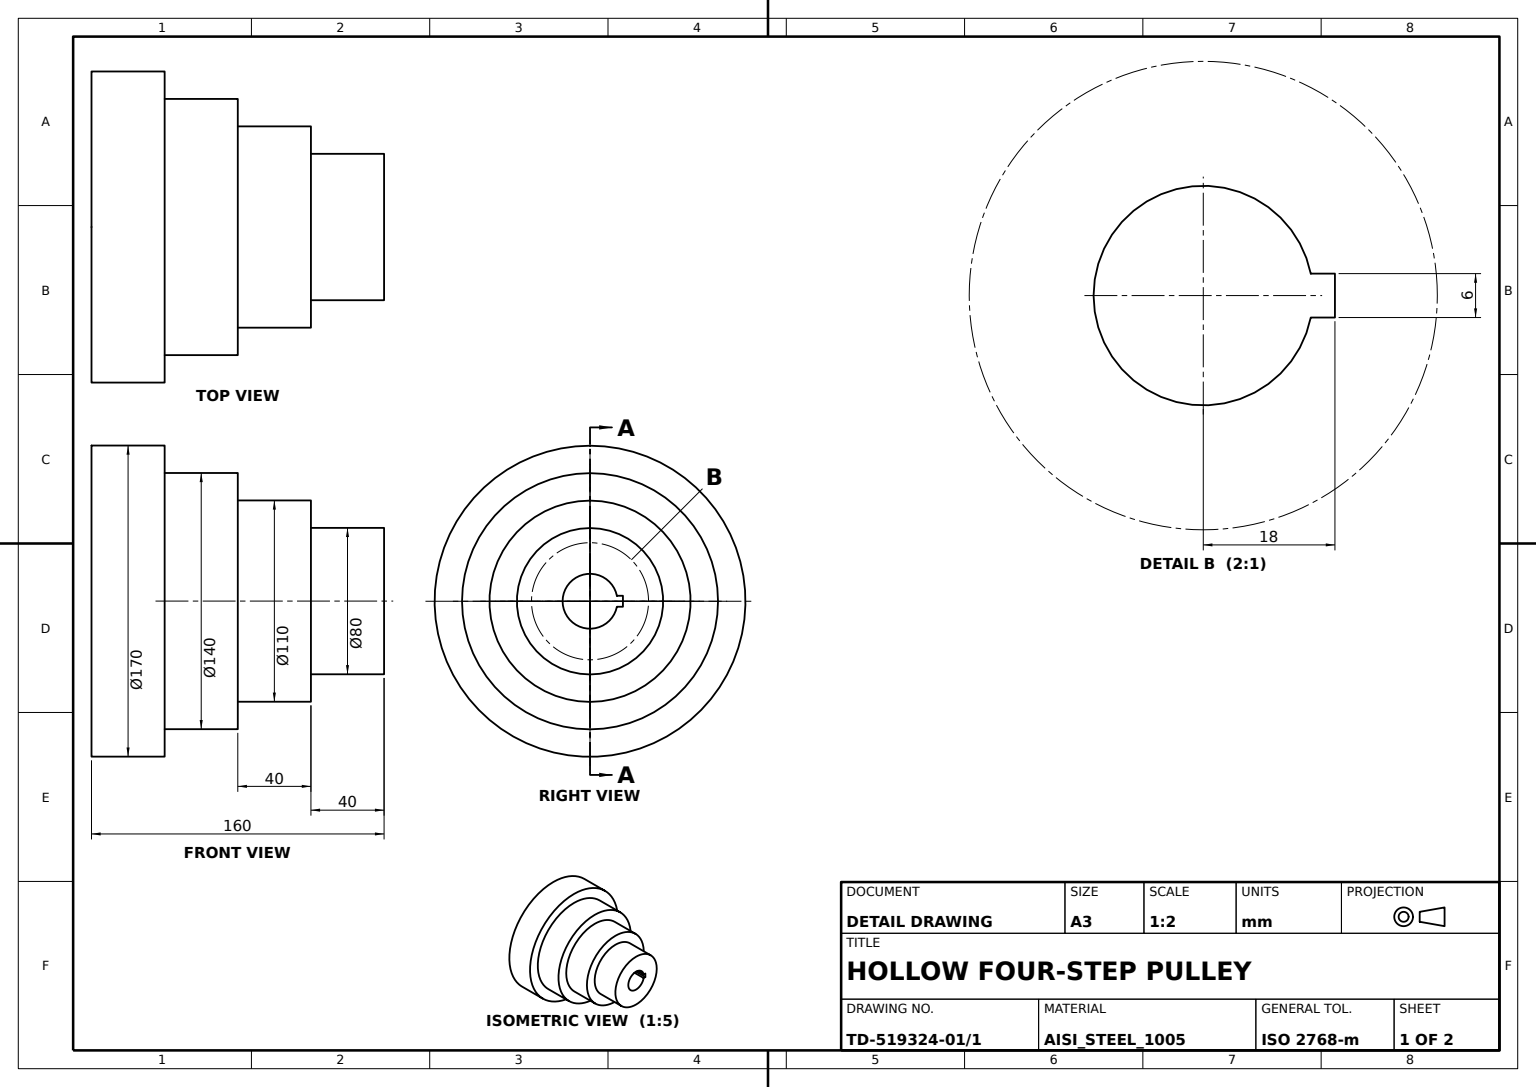
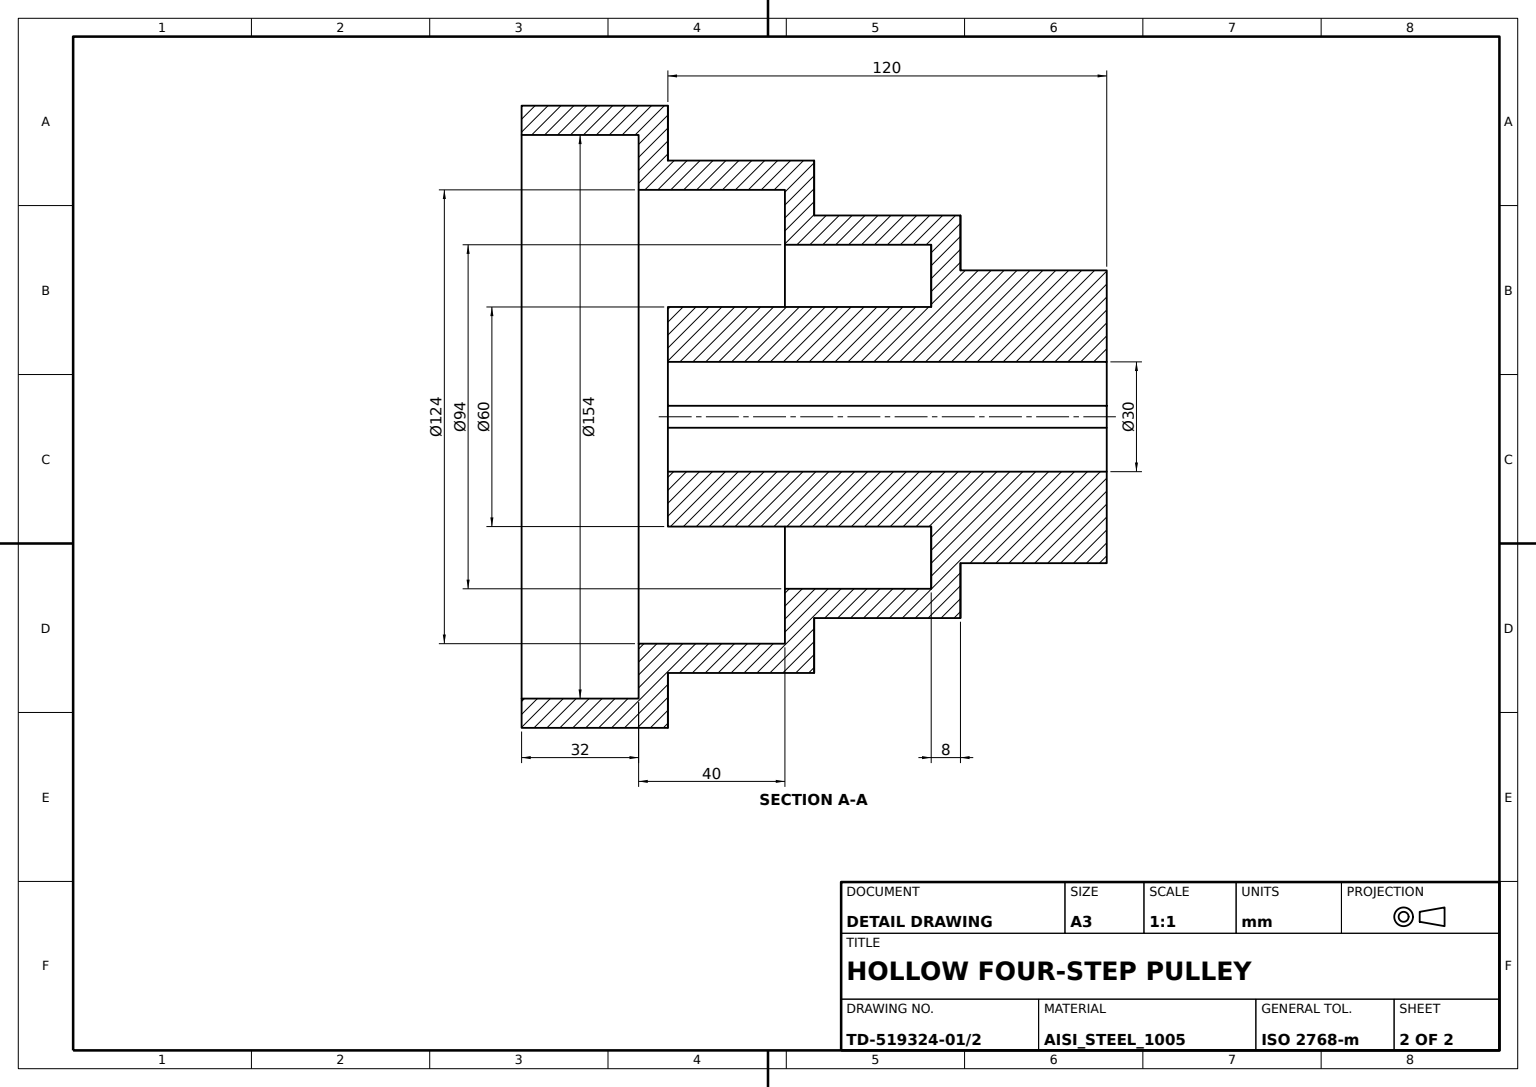
ISO-10303-21;
HEADER;
FILE_DESCRIPTION((''),'2;1');
FILE_NAME('','',(''),(''),'','','');
FILE_SCHEMA(('AUTOMOTIVE_DESIGN'));
ENDSEC;
DATA;
#1=APPLICATION_CONTEXT('');
#2=PRODUCT_CONTEXT('',#1,'mechanical');
#3=PRODUCT('','','',(#2));
#4=PRODUCT_DEFINITION_FORMATION('','',#3);
#5=PRODUCT_DEFINITION_CONTEXT('',#1,'design');
#6=PRODUCT_DEFINITION('','',#4,#5);
#7=PRODUCT_DEFINITION_SHAPE('','',#6);
#8=(LENGTH_UNIT()NAMED_UNIT(*)SI_UNIT(.MILLI.,.METRE.));
#9=(NAMED_UNIT(*)PLANE_ANGLE_UNIT()SI_UNIT($,.RADIAN.));
#10=(NAMED_UNIT(*)SI_UNIT($,.STERADIAN.)SOLID_ANGLE_UNIT());
#11=UNCERTAINTY_MEASURE_WITH_UNIT(LENGTH_MEASURE(0.005),#8,'distance_accuracy_value','');
#12=(GEOMETRIC_REPRESENTATION_CONTEXT(3)GLOBAL_UNCERTAINTY_ASSIGNED_CONTEXT((#11))GLOBAL_UNIT_ASSIGNED_CONTEXT((#8,#9,#10))REPRESENTATION_CONTEXT('',''));
#13=CARTESIAN_POINT('',(0.,72.,62.));
#14=VERTEX_POINT('',#13);
#15=CARTESIAN_POINT('',(0.,72.,0.));
#16=DIRECTION('',(0.,1.,0.));
#17=DIRECTION('',(0.,0.,1.));
#18=AXIS2_PLACEMENT_3D('',#15,#16,#17);
#19=CIRCLE('',#18,62.);
#20=EDGE_CURVE('',#14,#14,#19,.T.);
#21=ORIENTED_EDGE('',*,*,#20,.F.);
#22=EDGE_LOOP('',(#21));
#23=FACE_BOUND('',#22,.T.);
#24=CARTESIAN_POINT('',(0.,72.,47.));
#25=VERTEX_POINT('',#24);
#26=CIRCLE('',#18,47.);
#27=EDGE_CURVE('',#25,#25,#26,.T.);
#28=ORIENTED_EDGE('',*,*,#27,.T.);
#29=EDGE_LOOP('',(#28));
#30=FACE_BOUND('',#29,.T.);
#31=CARTESIAN_POINT('',(47.,72.,0.));
#32=AXIS2_PLACEMENT_3D('',#31,#16,#17);
#33=PLANE('',#32);
#34=ADVANCED_FACE('',(#23,#30),#33,.F.);
#35=CARTESIAN_POINT('',(0.,40.,70.));
#36=VERTEX_POINT('',#35);
#37=CARTESIAN_POINT('',(0.,40.,0.));
#38=AXIS2_PLACEMENT_3D('',#37,#16,#17);
#39=CIRCLE('',#38,70.);
#40=EDGE_CURVE('',#36,#36,#39,.T.);
#41=ORIENTED_EDGE('',*,*,#40,.T.);
#42=EDGE_LOOP('',(#41));
#43=FACE_BOUND('',#42,.T.);
#44=CARTESIAN_POINT('',(0.,80.,70.));
#45=VERTEX_POINT('',#44);
#46=CARTESIAN_POINT('',(0.,80.,0.));
#47=AXIS2_PLACEMENT_3D('',#46,#16,#17);
#48=CIRCLE('',#47,70.);
#49=EDGE_CURVE('',#45,#45,#48,.T.);
#50=ORIENTED_EDGE('',*,*,#49,.F.);
#51=EDGE_LOOP('',(#50));
#52=FACE_BOUND('',#51,.T.);
#53=CARTESIAN_POINT('',(0.,0.,0.));
#54=AXIS2_PLACEMENT_3D('',#53,#16,#17);
#55=CYLINDRICAL_SURFACE('',#54,70.);
#56=ADVANCED_FACE('',(#43,#52),#55,.T.);
#57=CARTESIAN_POINT('',(-18.,40.,-3.));
#58=VERTEX_POINT('',#57);
#59=CARTESIAN_POINT('',(-18.,40.,3.));
#60=VERTEX_POINT('',#59);
#61=VECTOR('',#17,1000.);
#62=LINE('',#59,#61);
#63=EDGE_CURVE('',#58,#60,#62,.T.);
#64=ORIENTED_EDGE('',*,*,#63,.F.);
#65=CARTESIAN_POINT('',(-18.,160.,-3.));
#66=VERTEX_POINT('',#65);
#67=CARTESIAN_POINT('',(-18.,-54840.,-3.));
#68=VECTOR('',#16,1000.);
#69=LINE('',#67,#68);
#70=EDGE_CURVE('',#66,#58,#69,.F.);
#71=ORIENTED_EDGE('',*,*,#70,.F.);
#72=CARTESIAN_POINT('',(-18.,160.,3.));
#73=VERTEX_POINT('',#72);
#74=DIRECTION('',(0.,0.,-1.));
#75=VECTOR('',#74,1000.);
#76=LINE('',#72,#75);
#77=EDGE_CURVE('',#73,#66,#76,.T.);
#78=ORIENTED_EDGE('',*,*,#77,.F.);
#79=CARTESIAN_POINT('',(-18.,-54840.,3.));
#80=LINE('',#79,#68);
#81=EDGE_CURVE('',#73,#60,#80,.F.);
#82=ORIENTED_EDGE('',*,*,#81,.T.);
#83=EDGE_LOOP('',(#64,#71,#78,#82));
#84=FACE_BOUND('',#83,.T.);
#85=DIRECTION('',(1.,0.,0.));
#86=AXIS2_PLACEMENT_3D('',#79,#85,#74);
#87=PLANE('',#86);
#88=ADVANCED_FACE('',(#84),#87,.T.);
#89=CARTESIAN_POINT('',(-14.696938,40.,3.));
#90=VERTEX_POINT('',#89);
#91=VECTOR('',#85,1000.);
#92=LINE('',#89,#91);
#93=EDGE_CURVE('',#60,#90,#92,.T.);
#94=ORIENTED_EDGE('',*,*,#93,.F.);
#95=ORIENTED_EDGE('',*,*,#81,.F.);
#96=CARTESIAN_POINT('',(-14.696938,160.,3.));
#97=VERTEX_POINT('',#96);
#98=DIRECTION('',(-1.,0.,0.));
#99=VECTOR('',#98,1000.);
#100=LINE('',#96,#99);
#101=EDGE_CURVE('',#97,#73,#100,.T.);
#102=ORIENTED_EDGE('',*,*,#101,.F.);
#103=CARTESIAN_POINT('',(-14.696938,-54840.,3.));
#104=LINE('',#103,#68);
#105=EDGE_CURVE('',#90,#97,#104,.T.);
#106=ORIENTED_EDGE('',*,*,#105,.F.);
#107=EDGE_LOOP('',(#94,#95,#102,#106));
#108=FACE_BOUND('',#107,.T.);
#109=AXIS2_PLACEMENT_3D('',#103,#74,#98);
#110=PLANE('',#109);
#111=ADVANCED_FACE('',(#108),#110,.T.);
#112=CARTESIAN_POINT('',(-14.696938,40.,-3.));
#113=VERTEX_POINT('',#112);
#114=LINE('',#57,#99);
#115=EDGE_CURVE('',#113,#58,#114,.T.);
#116=ORIENTED_EDGE('',*,*,#115,.F.);
#117=CARTESIAN_POINT('',(-14.696938,160.,-3.));
#118=VERTEX_POINT('',#117);
#119=CARTESIAN_POINT('',(-14.696938,-54840.,-3.));
#120=LINE('',#119,#68);
#121=EDGE_CURVE('',#113,#118,#120,.T.);
#122=ORIENTED_EDGE('',*,*,#121,.T.);
#123=LINE('',#65,#91);
#124=EDGE_CURVE('',#66,#118,#123,.T.);
#125=ORIENTED_EDGE('',*,*,#124,.F.);
#126=ORIENTED_EDGE('',*,*,#70,.T.);
#127=EDGE_LOOP('',(#116,#122,#125,#126));
#128=FACE_BOUND('',#127,.T.);
#129=AXIS2_PLACEMENT_3D('',#67,#17,#85);
#130=PLANE('',#129);
#131=ADVANCED_FACE('',(#128),#130,.T.);
#132=CARTESIAN_POINT('',(0.,32.,77.));
#133=VERTEX_POINT('',#132);
#134=CARTESIAN_POINT('',(0.,32.,0.));
#135=AXIS2_PLACEMENT_3D('',#134,#16,#17);
#136=CIRCLE('',#135,77.);
#137=EDGE_CURVE('',#133,#133,#136,.T.);
#138=ORIENTED_EDGE('',*,*,#137,.F.);
#139=EDGE_LOOP('',(#138));
#140=FACE_BOUND('',#139,.T.);
#141=CARTESIAN_POINT('',(0.,32.,62.));
#142=VERTEX_POINT('',#141);
#143=CIRCLE('',#135,62.);
#144=EDGE_CURVE('',#142,#142,#143,.T.);
#145=ORIENTED_EDGE('',*,*,#144,.T.);
#146=EDGE_LOOP('',(#145));
#147=FACE_BOUND('',#146,.T.);
#148=CARTESIAN_POINT('',(62.,32.,0.));
#149=AXIS2_PLACEMENT_3D('',#148,#16,#17);
#150=PLANE('',#149);
#151=ADVANCED_FACE('',(#140,#147),#150,.F.);
#152=CARTESIAN_POINT('',(0.,0.,85.));
#153=VERTEX_POINT('',#152);
#154=CIRCLE('',#54,85.);
#155=EDGE_CURVE('',#153,#153,#154,.T.);
#156=ORIENTED_EDGE('',*,*,#155,.F.);
#157=EDGE_LOOP('',(#156));
#158=FACE_BOUND('',#157,.T.);
#159=CARTESIAN_POINT('',(0.,0.,77.));
#160=VERTEX_POINT('',#159);
#161=CIRCLE('',#54,77.);
#162=EDGE_CURVE('',#160,#160,#161,.T.);
#163=ORIENTED_EDGE('',*,*,#162,.T.);
#164=EDGE_LOOP('',(#163));
#165=FACE_BOUND('',#164,.T.);
#166=CARTESIAN_POINT('',(77.,0.,0.));
#167=AXIS2_PLACEMENT_3D('',#166,#16,#17);
#168=PLANE('',#167);
#169=ADVANCED_FACE('',(#158,#165),#168,.F.);
#170=ORIENTED_EDGE('',*,*,#20,.T.);
#171=EDGE_LOOP('',(#170));
#172=FACE_BOUND('',#171,.T.);
#173=ORIENTED_EDGE('',*,*,#144,.F.);
#174=EDGE_LOOP('',(#173));
#175=FACE_BOUND('',#174,.T.);
#176=CYLINDRICAL_SURFACE('',#54,62.);
#177=ADVANCED_FACE('',(#172,#175),#176,.F.);
#178=CARTESIAN_POINT('',(0.,160.,40.));
#179=VERTEX_POINT('',#178);
#180=CARTESIAN_POINT('',(0.,160.,0.));
#181=AXIS2_PLACEMENT_3D('',#180,#16,#17);
#182=CIRCLE('',#181,40.);
#183=EDGE_CURVE('',#179,#179,#182,.T.);
#184=ORIENTED_EDGE('',*,*,#183,.F.);
#185=EDGE_LOOP('',(#184));
#186=FACE_BOUND('',#185,.T.);
#187=CARTESIAN_POINT('',(0.,120.,40.));
#188=VERTEX_POINT('',#187);
#189=CARTESIAN_POINT('',(0.,120.,0.));
#190=AXIS2_PLACEMENT_3D('',#189,#16,#17);
#191=CIRCLE('',#190,40.);
#192=EDGE_CURVE('',#188,#188,#191,.T.);
#193=ORIENTED_EDGE('',*,*,#192,.T.);
#194=EDGE_LOOP('',(#193));
#195=FACE_BOUND('',#194,.T.);
#196=CYLINDRICAL_SURFACE('',#54,40.);
#197=ADVANCED_FACE('',(#186,#195),#196,.T.);
#198=CARTESIAN_POINT('',(0.,120.,55.));
#199=VERTEX_POINT('',#198);
#200=CIRCLE('',#190,55.);
#201=EDGE_CURVE('',#199,#199,#200,.T.);
#202=ORIENTED_EDGE('',*,*,#201,.T.);
#203=EDGE_LOOP('',(#202));
#204=FACE_BOUND('',#203,.T.);
#205=ORIENTED_EDGE('',*,*,#192,.F.);
#206=EDGE_LOOP('',(#205));
#207=FACE_BOUND('',#206,.T.);
#208=CARTESIAN_POINT('',(55.,120.,0.));
#209=DIRECTION('',(0.,-1.,0.));
#210=AXIS2_PLACEMENT_3D('',#208,#209,#74);
#211=PLANE('',#210);
#212=ADVANCED_FACE('',(#204,#207),#211,.F.);
#213=CARTESIAN_POINT('',(0.,112.,47.));
#214=VERTEX_POINT('',#213);
#215=CARTESIAN_POINT('',(0.,112.,0.));
#216=AXIS2_PLACEMENT_3D('',#215,#16,#17);
#217=CIRCLE('',#216,47.);
#218=EDGE_CURVE('',#214,#214,#217,.T.);
#219=ORIENTED_EDGE('',*,*,#218,.T.);
#220=EDGE_LOOP('',(#219));
#221=FACE_BOUND('',#220,.T.);
#222=ORIENTED_EDGE('',*,*,#27,.F.);
#223=EDGE_LOOP('',(#222));
#224=FACE_BOUND('',#223,.T.);
#225=CYLINDRICAL_SURFACE('',#54,47.);
#226=ADVANCED_FACE('',(#221,#224),#225,.F.);
#227=ORIENTED_EDGE('',*,*,#201,.F.);
#228=EDGE_LOOP('',(#227));
#229=FACE_BOUND('',#228,.T.);
#230=CARTESIAN_POINT('',(0.,80.,55.));
#231=VERTEX_POINT('',#230);
#232=CIRCLE('',#47,55.);
#233=EDGE_CURVE('',#231,#231,#232,.T.);
#234=ORIENTED_EDGE('',*,*,#233,.T.);
#235=EDGE_LOOP('',(#234));
#236=FACE_BOUND('',#235,.T.);
#237=CYLINDRICAL_SURFACE('',#54,55.);
#238=ADVANCED_FACE('',(#229,#236),#237,.T.);
#239=ORIENTED_EDGE('',*,*,#155,.T.);
#240=EDGE_LOOP('',(#239));
#241=FACE_BOUND('',#240,.T.);
#242=CARTESIAN_POINT('',(0.,40.,85.));
#243=VERTEX_POINT('',#242);
#244=CIRCLE('',#38,85.);
#245=EDGE_CURVE('',#243,#243,#244,.T.);
#246=ORIENTED_EDGE('',*,*,#245,.F.);
#247=EDGE_LOOP('',(#246));
#248=FACE_BOUND('',#247,.T.);
#249=CYLINDRICAL_SURFACE('',#54,85.);
#250=ADVANCED_FACE('',(#241,#248),#249,.T.);
#251=ORIENTED_EDGE('',*,*,#77,.T.);
#252=ORIENTED_EDGE('',*,*,#124,.T.);
#253=CIRCLE('',#181,15.);
#254=EDGE_CURVE('',#97,#118,#253,.T.);
#255=ORIENTED_EDGE('',*,*,#254,.F.);
#256=ORIENTED_EDGE('',*,*,#101,.T.);
#257=EDGE_LOOP('',(#251,#252,#255,#256));
#258=FACE_BOUND('',#257,.T.);
#259=ORIENTED_EDGE('',*,*,#183,.T.);
#260=EDGE_LOOP('',(#259));
#261=FACE_BOUND('',#260,.T.);
#262=CARTESIAN_POINT('',(40.,160.,0.));
#263=AXIS2_PLACEMENT_3D('',#262,#209,#74);
#264=PLANE('',#263);
#265=ADVANCED_FACE('',(#258,#261),#264,.F.);
#266=CARTESIAN_POINT('',(0.,112.,30.));
#267=VERTEX_POINT('',#266);
#268=CIRCLE('',#216,30.);
#269=EDGE_CURVE('',#267,#267,#268,.T.);
#270=ORIENTED_EDGE('',*,*,#269,.T.);
#271=EDGE_LOOP('',(#270));
#272=FACE_BOUND('',#271,.T.);
#273=ORIENTED_EDGE('',*,*,#218,.F.);
#274=EDGE_LOOP('',(#273));
#275=FACE_BOUND('',#274,.T.);
#276=CARTESIAN_POINT('',(30.,112.,0.));
#277=AXIS2_PLACEMENT_3D('',#276,#16,#17);
#278=PLANE('',#277);
#279=ADVANCED_FACE('',(#272,#275),#278,.F.);
#280=ORIENTED_EDGE('',*,*,#233,.F.);
#281=EDGE_LOOP('',(#280));
#282=FACE_BOUND('',#281,.T.);
#283=ORIENTED_EDGE('',*,*,#49,.T.);
#284=EDGE_LOOP('',(#283));
#285=FACE_BOUND('',#284,.T.);
#286=CARTESIAN_POINT('',(70.,80.,0.));
#287=AXIS2_PLACEMENT_3D('',#286,#209,#74);
#288=PLANE('',#287);
#289=ADVANCED_FACE('',(#282,#285),#288,.F.);
#290=CARTESIAN_POINT('',(0.,40.,30.));
#291=VERTEX_POINT('',#290);
#292=CIRCLE('',#38,30.);
#293=EDGE_CURVE('',#291,#291,#292,.T.);
#294=ORIENTED_EDGE('',*,*,#293,.T.);
#295=EDGE_LOOP('',(#294));
#296=FACE_BOUND('',#295,.T.);
#297=ORIENTED_EDGE('',*,*,#269,.F.);
#298=EDGE_LOOP('',(#297));
#299=FACE_BOUND('',#298,.T.);
#300=CYLINDRICAL_SURFACE('',#54,30.);
#301=ADVANCED_FACE('',(#296,#299),#300,.T.);
#302=ORIENTED_EDGE('',*,*,#254,.T.);
#303=ORIENTED_EDGE('',*,*,#121,.F.);
#304=CIRCLE('',#38,15.);
#305=EDGE_CURVE('',#90,#113,#304,.T.);
#306=ORIENTED_EDGE('',*,*,#305,.F.);
#307=ORIENTED_EDGE('',*,*,#105,.T.);
#308=EDGE_LOOP('',(#302,#303,#306,#307));
#309=FACE_BOUND('',#308,.T.);
#310=CYLINDRICAL_SURFACE('',#54,15.);
#311=ADVANCED_FACE('',(#309),#310,.F.);
#312=ORIENTED_EDGE('',*,*,#293,.F.);
#313=EDGE_LOOP('',(#312));
#314=FACE_BOUND('',#313,.T.);
#315=ORIENTED_EDGE('',*,*,#305,.T.);
#316=ORIENTED_EDGE('',*,*,#115,.T.);
#317=ORIENTED_EDGE('',*,*,#63,.T.);
#318=ORIENTED_EDGE('',*,*,#93,.T.);
#319=EDGE_LOOP('',(#315,#316,#317,#318));
#320=FACE_BOUND('',#319,.T.);
#321=CARTESIAN_POINT('',(15.,40.,0.));
#322=AXIS2_PLACEMENT_3D('',#321,#16,#17);
#323=PLANE('',#322);
#324=ADVANCED_FACE('',(#314,#320),#323,.F.);
#325=ORIENTED_EDGE('',*,*,#245,.T.);
#326=EDGE_LOOP('',(#325));
#327=FACE_BOUND('',#326,.T.);
#328=ORIENTED_EDGE('',*,*,#40,.F.);
#329=EDGE_LOOP('',(#328));
#330=FACE_BOUND('',#329,.T.);
#331=CARTESIAN_POINT('',(85.,40.,0.));
#332=AXIS2_PLACEMENT_3D('',#331,#209,#74);
#333=PLANE('',#332);
#334=ADVANCED_FACE('',(#327,#330),#333,.F.);
#335=ORIENTED_EDGE('',*,*,#137,.T.);
#336=EDGE_LOOP('',(#335));
#337=FACE_BOUND('',#336,.T.);
#338=ORIENTED_EDGE('',*,*,#162,.F.);
#339=EDGE_LOOP('',(#338));
#340=FACE_BOUND('',#339,.T.);
#341=CYLINDRICAL_SURFACE('',#54,77.);
#342=ADVANCED_FACE('',(#337,#340),#341,.F.);
#343=CLOSED_SHELL('',(#34,#56,#88,#111,#131,#151,#169,#177,#197,#212,#226,#238,#250,#265,#279,#289,#301,#311,#324,#334,#342));
#344=MANIFOLD_SOLID_BREP('',#343);
#345=ADVANCED_BREP_SHAPE_REPRESENTATION('',(#344),#12);
#346=SHAPE_DEFINITION_REPRESENTATION(#7,#345);
ENDSEC;
END-ISO-10303-21;
